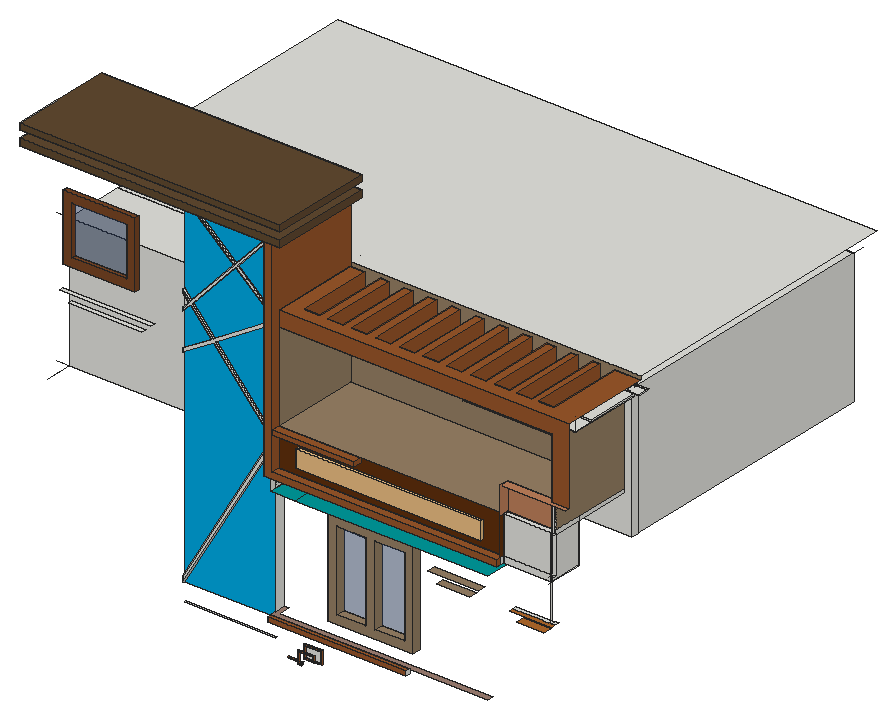
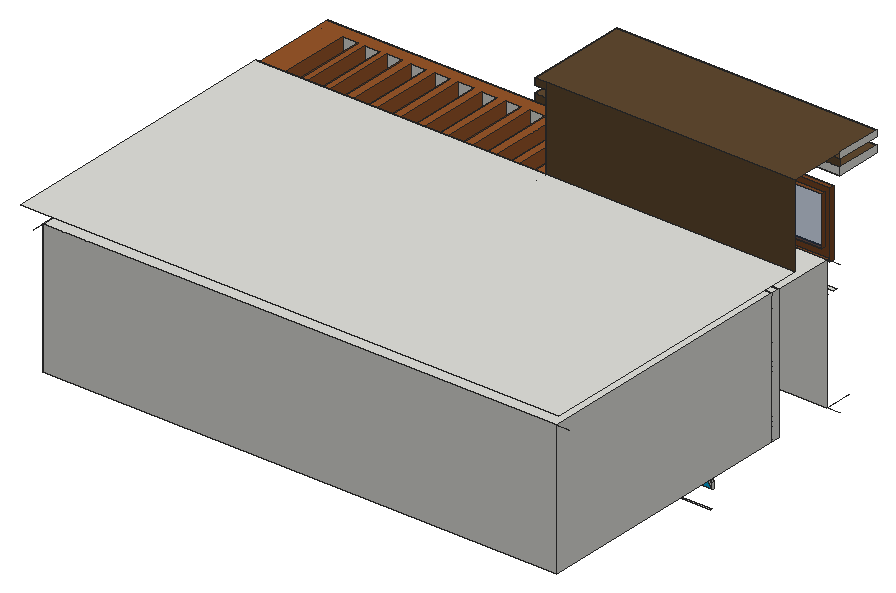
# SketchUp Ruby script. Lengths in inches.
U = 1.inch
M = Sketchup.active_model
def pt(a) = Geom::Point3d.new(a.map { |v| v * U })
def face(e, loops, mat)
  f = e.add_face(loops[0].map { |a| pt(a) })
  loops[1..].each { |l| e.add_face(l.map { |a| pt(a) }).erase! }
  f.material = f.back_material = mat if mat
  f
end
# faces: each face lists its corners as indices into pts; further lists are holes
def faces(e, pts, list, mat = nil) = list.each { |f| face(e, (f[0].is_a?(Array) ? f : [f]).map { |l| l.map { |i| pts[i] } }, mat) }
# xy, xz, yz: faces in a plane at the given z, y or x. An outline is a flat list of corners, or four numbers for a rectangle; further outlines are holes
def ring(l) = l.size == 4 ? [[l[0], l[1]], [l[2], l[1]], [l[2], l[3]], [l[0], l[3]]] : l.each_slice(2).to_a
def flat(e, list, mat, &to3) = list.each { |f| face(e, (f[0].is_a?(Array) ? f : [f]).map { |l| ring(l).map { |u, v| to3.(u, v) } }, mat) }
def xy(e, z, list, mat = nil) = flat(e, list, mat) { |x, y| [x, y, z] }
def xz(e, y, list, mat = nil) = flat(e, list, mat) { |x, z| [x, y, z] }
def yz(e, x, list, mat = nil) = flat(e, list, mat) { |y, z| [x, y, z] }
def lines(e, pts, list) = list.each { |a, b| e.add_line(pt(pts[a]), pt(pts[b])) }
# prism: a flat outline (further loops are holes) pulled along v
def prism(e, loops, v, mat = nil)
  f = face(e, loops, mat); d = Geom::Vector3d.new(v.map { |x| x * U })
  f.pushpull(f.normal.samedirection?(d) ? d.length : -d.length)
end
def box(e, o, s, mat = nil) = prism(e, [[o, [o[0] + s[0], o[1], o[2]], [o[0] + s[0], o[1] + s[1], o[2]], [o[0], o[1] + s[1], o[2]]]], [0, 0, s[2]], mat)
def at(x, y, z, deg = 0) = Geom::Transformation.translation(pt([x, y, z])) * Geom::Transformation.rotation(ORIGIN, Z_AXIS, deg.degrees)
def axes(o, x, y, z) = Geom::Transformation.new([*x, 0, *y, 0, *z, 0, *pt(o).to_a, 1])
def part(name) = M.definitions.add(name)
# library, detail: a bought-in or finely detailed component or shape, given as its bounding box
def library(name, o, s) = part(name).tap { |d| box(d.entities, o, s) }
def detail(e, o, s) = box(e.add_group.entities, o, s)
def put(e, d, t, mat = nil) = e.add_instance(d, t).tap { |i| i.material = mat if mat }
def group(e, t, mat = nil) = e.add_group.tap { |g| g.transformation = t; g.material = mat if mat }.entities
root = M.entities
M.materials.add("Niraj_Shoe_Sole").color = [96, 73, 48]
M.materials.add("Niraj_Skin").color = [158, 128, 115]
M.materials.add("[0035_Tan]").color = [150, 128, 100]
M.materials.add("[0043_SaddleBrown]").color = [96, 48, 13]
M.materials.add("[0083_DarkTurquoise]").color = [0, 153, 155]
M.materials.add("[0097_DeepSkyBlue]").color = [0, 169, 226]
M.materials.add("[0097_DeepSkyBlue]1").color = [0, 171, 229]
M.materials.add("[Basketweave]").color = [230, 230, 230]
M.materials.add("[Translucent Glass Blue]").color = [40, 60, 96]
M.materials["[Translucent Glass Blue]"].alpha = 0.5
M.materials.add("[Wood Bamboo]").color = [177, 105, 43]
M.materials.add("[Wood Cherry Original]").color = [152, 86, 42]
M.materials.add("[Wood Veneer 01]").color = [120, 70, 37]
M.materials.add("[Wood Veneer 02]").color = [190, 128, 91]
c1 = library("NAKSHA MART",[0.95,0,0],[104.73,9.95,1])
xy(root,148.76,[[191.85,117,194.8,118]],"[Wood Cherry Original]")
xy(root,149.21,[[192.49,117,194.8,118]],"[Wood Cherry Original]")
xy(root,150.16,[[185.22,117,191.85,118],[192.49,117,194.8,118]],"[Wood Cherry Original]")
xy(root,150.73,[[184.65,117,191.85,118],[192.49,117,195.37,118]],"[Wood Cherry Original]")
xy(root,153.79,[[196.34,117,203.17,118],[203.17,117,208.53,118]],"[Wood Cherry Original]")
xy(root,154.4,[[196.95,117,202.56,118],[203.17,117,207.92,118]],"[Wood Cherry Original]")
xy(root,156.27,[[106.63,122.375,171.63,123.3125]])
xy(root,157.02,[[192.49,117,196.95,118],[196.95,117,202.56,118]],"[Wood Cherry Original]")
xy(root,157.63,[[191.85,117,196.34,118],[196.95,117,203.17,118]],"[Wood Cherry Original]")
xy(root,162.4375,[[196.95,117,207.92,118]],"[Wood Cherry Original]")
xy(root,163.04,[[196.34,117,208.53,118]],"[Wood Cherry Original]")
xy(root,169.5625,[[171.63,115,270.57,118]],"[Wood Cherry Original]")
xy(root,170.25,[[198.26,136,258.45,142]])
xy(root,172.875,[[171.63,118,326.57,118,326.57,122.125,175.07,122.125,175.07,130,171.63,130]],"Niraj_Skin")
xy(root,172.875,[[171.63,115,270.57,118]],"[Wood Cherry Original]")
xy(root,176.25,[[204.26,136,225.35,142],[231.35,136,252.45,142]],"[0035_Tan]")
xy(root,220.875,[[275.26,136,299.26,142]],"[0035_Tan]")
xy(root,226.875,[[269.26,136,305.26,142]],"[0035_Tan]")
xy(root,233,[[204.26,136,225.35,142],[231.35,136,252.45,142]],"[0035_Tan]")
xy(root,233.83,[[351.89,112,371.22,118]],"[Wood Bamboo]")
xy(root,239,[[198.26,136,258.45,142]],"[0035_Tan]")
xy(root,239.26,[[346.46,115,372,118],[372,115,374.5,118],[374.5,115,376.65,118]])
xy(root,239.26,[[346.46,112,376.65,115]],"[Wood Bamboo]")
xy(root,251.8,[[171.63,130,189.04,142]])
xy(root,251.8,[[171.63,118,189.04,130],[189.04,118,326.57,142]],"[0083_DarkTurquoise]")
xy(root,264,[[171.63,118,337.38,142],[337.38,118,337.94,142],[337.94,118,371.25,142],[371.25,118,372,142],[9,185.375,375,190.9375],
  [9,190.9375,375,191.0625]])
xy(root,264,[[171.63,112,337.38,118]],"[Wood Cherry Original]")
xy(root,268.5,[[177.19,112,337.38,118]],"[Wood Cherry Original]")
xy(root,292.26,[[177.19,112,236,118]],"[Wood Cherry Original]")
xy(root,292.65,[[337.38,121.62,337.94,142],[371.25,121.62,371.25,142,337.38,142,337.38,182.0625,372,182.0625,372,121.62],[337.94,121.62,371.25,142]])
xy(root,295.34,[[337.38,118,337.94,121.62],[337.94,118,371.25,121.62],[371.25,118,372,121.62]])
xy(root,295.34,[[177.19,118,337.38,118,337.38,121.62,372,121.62,372,182.0625,177.19,182.0625]],"[0035_Tan]")
xy(root,295.34,[[177.19,112,236,118]],"[Wood Cherry Original]")
xy(root,310.87,[[257.29,182.0625,340.41,185.375]])
xy(root,314.9,[[337.38,115,384,115,384,118,372,118,372,121.62,337.38,121.62]],"[Wood Veneer 02]")
xy(root,319.95,[[26.53,119.375,78.96,122.375]])
xy(root,326.3125,[[20.16,119.375,85.33,122.375]])
xy(root,343.6,[[22.76,119.375,74.01,122.375]],"[Wood Veneer 01]")
xy(root,348.68,[[257.29,182.0625,340.41,185.375]])
xy(root,349.76,[[28.92,119.375,67.85,122.375]],"[Wood Veneer 01]")
xy(root,358.625,[[372,127.53,381.34,142],[372,127.53,381.34,179.66],[9,142,177.19,185.375],[372,182.0625,375,185.375],[375,182.0625,382.75,189.21],
  [9,185.375,177.19,190.9375],[177.19,185.375,177.19,190.9375,373.3125,190.9375,373.3125,189.21,372,189.21,372,185.375],[372,185.375,375,189.21],[373.3125,189.21,375,190.9375],[375,189.21,382.75,191.0625],
  [9,190.9375,177.19,191.0625],[177.19,190.9375,372,191.0625],[372,190.9375,373.3125,191.0625],[373.3125,190.9375,375,191.0625],[9,191.0625,9,382.875,375,382.875,375,191.0625,372,191.0625,372,191.1875,177.19,191.1875,177.19,191.0625],
  [177.19,191.0625,372,191.1875]])
xy(root,358.625,[[177.19,118,177.19,181.83,187.9,181.83,187.9,127.72,198.78,127.72,198.78,181.83,204.84,181.83,204.84,127.53,215.72,127.53,215.72,181.83,221.78,181.83,221.78,127.53,232.65,127.53,232.65,181.83,238.72,181.83,238.72,127.53,249.59,127.53,249.59,181.83,255.65,181.83,255.65,127.53,266.53,127.53,266.53,181.83,272.59,181.83,272.59,127.53,283.47,127.53,283.47,181.83,289.53,181.83,289.53,127.53,300.4,127.53,300.4,181.83,306.47,181.83,306.47,127.53,317.34,127.53,317.34,181.83,323.4,181.83,323.4,127.53,334.28,127.53,334.28,181.83,339.09,181.83,339.09,127.53,349.97,127.53,349.97,181.83,354.78,181.83,354.78,127.53,365.65,127.53,365.65,181.83,372,181.83,372,118]],"[Wood Cherry Original]")
xy(root,358.9375,[[370.47,127.53,381.34,179.66],[365.65,181.83,372,190.89],[372,182.0625,373.3125,189.21]])
xy(root,359.1875,[[171.63,118,177.19,142],[373.3125,182.0625,382.75,189.21]])
xy(root,359.625,[[370.47,127.53,372,179.66]])
xy(root,360.375,[[372,142,381.34,179.66]])
xy(root,361.5,[[171.63,118,177.19,142]])
xy(root,369.0625,[[177.19,118,384,118,384,182.0625,375,182.0625,375,181.83,365.65,181.83,365.65,127.53,354.78,127.53,354.78,181.83,349.97,181.83,349.97,127.53,339.09,127.53,339.09,181.83,334.28,181.83,334.28,127.53,323.4,127.53,323.4,181.83,317.34,181.83,317.34,127.53,306.47,127.53,306.47,181.83,300.4,181.83,300.4,127.53,289.53,127.53,289.53,181.83,283.47,181.83,283.47,127.53,272.59,127.53,272.59,181.83,266.53,181.83,266.53,127.53,255.65,127.53,255.65,181.83,249.59,181.83,249.59,127.53,238.72,127.53,238.72,181.83,232.65,181.83,232.65,127.53,221.78,127.53,221.78,181.83,215.72,181.83,215.72,127.53,204.84,127.53,204.84,181.83,198.78,181.83,198.78,127.72,187.9,127.72,187.9,181.83,177.19,181.83]],"[Wood Cherry Original]")
xy(root,371.75,[[0,182.0625,384,391.875]])
xy(root,384.9375,[[28.92,119.375,67.85,122.375]],"[Wood Veneer 01]")
xy(root,391.1,[[22.76,119.375,74.01,122.375]],"[Wood Veneer 01]")
xy(root,415.46,[[171.63,112,177.19,118],[171.63,118,177.19,142],[106.63,121.375,106.63,122.375,0,122.375,0,142,171.63,142,171.63,122.375,109.24,122.375,109.24,121.375]])
xy(root,415.46,[[0,109.5625,0,122.375,106.63,122.375,106.63,121.375,109.24,121.375,109.24,122.375,171.63,122.375,171.63,112,177.19,112,177.19,182.0625,185.19,182.0625,185.19,109.5625]],"Niraj_Shoe_Sole")
xy(root,420.59,[[0,109.5625,185.19,109.5625,185.19,182.0625,177.19,182.0625,177.19,142,0,142]],"Niraj_Shoe_Sole")
xy(root,425.72,[[0,109.5625,0,142,177.19,142,177.19,182.0625,185.19,182.0625,185.19,109.5625]],"Niraj_Shoe_Sole")
xy(root,430.21,[[0,109.5625,185.19,182.0625]],"Niraj_Shoe_Sole")
xz(root,109.5625,[[0,415.46,185.19,420.59],[0,425.72,185.19,430.21]],"Niraj_Shoe_Sole")
xz(root,112,[[171.63,264,337.38,264,337.38,268.5,177.19,268.5,177.19,415.46,171.63,415.46],[177.19,292.26,236,295.34]],"[Wood Cherry Original]")
xz(root,115,[[171.63,169.5625,270.57,172.875]],"[Wood Cherry Original]")
xz(root,117,[[191.85,150.73,192.49,150.73,192.49,157.02,202.56,157.02,202.56,154.4,196.95,154.4,196.95,157.02,196.34,157.01,196.34,153.79,203.17,153.79,203.17,157.63,191.85,157.63],[203.17,153.79,208.53,153.79,208.53,163.04,196.34,163.04,196.34,157.63,196.95,157.63,196.95,162.4375,207.92,162.4375,207.92,154.4,203.17,154.4]],"[Wood Cherry Original]")
xz(root,118,[[192.49,149.21,194.8,150.16],[196.95,154.4,202.56,157.02],[203.17,154.4,207.92,154.4,207.92,162.4375,196.95,162.4375,196.95,157.63,203.17,157.63],[171.63,169.5625,270.57,172.875],[371.25,239.26,372,264],
  [171.63,264,171.63,359.1875,177.19,359.1875,177.19,268.5,337.38,268.5,337.38,264],[337.38,264,337.94,268.5],[337.94,264,371.25,268.5],[371.25,264,372,268.5],[337.38,268.5,337.94,295.34],
  [337.94,268.5,371.25,295.34],[371.25,268.5,372,295.34],[372,268.5,374.5,295.34],[177.19,292.26,236,293.14],[177.19,293.14,236,295.34],
  [372,295.34,373.19,314.9],[171.63,359.1875,177.19,361.5]])
xz(root,118,[[177.19,268.5,337.38,268.5,337.38,295.34,236,295.34,236,292.26,177.19,292.26]],"[0043_SaddleBrown]")
xz(root,118,[[372,314.9,384,314.9,384,369.0625,177.19,369.0625,177.19,358.625,372,358.625]],"[Wood Cherry Original]")
xz(root,119.375,[[[22.76,343.6,74.01,391.1],[28.92,349.76,67.85,384.9375]]],"[Wood Veneer 01]")
xz(root,121.375,[[106.63,169.15,171.63,280.38,171.63,283.38,129.8125,330.53,171.63,356.59,171.63,359.1875,128.36,332.17,113.11,349.37,144.1,383.02,171.63,359.1875,171.63,361.5,145.27,384.3,171.63,412.93,171.63,415.46,144.03,385.37,109.24,415.46,106.63,415.46,142.86,384.09,112.08,350.53,106.63,356.67,106.63,353.72,110.75,349.07,106.63,344.58,106.63,342.33,111.77,347.92,126.66,331.12,106.63,318.61,106.63,316.08,128.12,329.47,169.73,282.52,106.63,173.48]])
xz(root,121.62,[[337.38,292.65,337.94,295.34],[337.94,292.65,371.25,295.34],[371.25,292.65,372,295.34]])
xz(root,121.62,[[337.38,295.34,372,314.9]],"[Wood Veneer 02]")
xz(root,122.375,[[106.63,344.58,110.75,349.07,106.63,353.72]])
xz(root,122.375,[[106.63,173.48,169.73,282.52,128.12,329.47,106.63,316.08],[171.63,283.38,171.63,356.59,129.8125,330.53],[106.63,318.61,126.66,331.12,111.77,347.92,106.63,342.33],[128.36,332.17,171.63,359.1875,144.1,383.02,113.11,349.37],[112.08,350.53,142.86,384.09,106.63,415.46,106.63,356.67],
  [171.63,361.5,171.63,412.93,145.27,384.3],[144.03,385.37,171.63,415.46,109.24,415.46]],"[0097_DeepSkyBlue]")
xz(root,122.375,[[106.63,169.15,171.63,169.15,171.63,280.38]],"[0097_DeepSkyBlue]1")
xz(root,122.375,[[28.92,349.76,67.85,384.9375]],"[Translucent Glass Blue]")
xz(root,127.53,[[204.84,358.625,215.72,358.9375],[221.78,358.625,232.65,358.9375],[238.72,358.625,249.59,358.9375],[255.65,358.625,266.53,358.9375],[272.59,358.625,283.47,358.9375],
  [289.53,358.625,300.4,358.9375],[306.47,358.625,317.34,358.9375],[323.4,358.625,334.28,358.9375],[339.09,358.625,349.97,358.9375],[354.78,358.625,365.65,358.9375],
  [372,358.625,381.34,358.9375],[204.84,358.9375,215.72,369.0625],[221.78,358.9375,232.65,369.0625],[238.72,358.9375,249.59,369.0625],[255.65,358.9375,266.53,369.0625],
  [272.59,358.9375,283.47,369.0625],[289.53,358.9375,300.4,369.0625],[306.47,358.9375,317.34,369.0625],[323.4,358.9375,334.28,369.0625],[339.09,358.9375,349.97,369.0625],
  [354.78,358.9375,365.65,369.0625],[370.47,358.9375,372,359.625]])
xz(root,127.72,[[187.9,358.625,198.78,358.9375],[187.9,358.9375,198.78,369.0625]])
xz(root,136,[[[198.26,170.25,258.45,239],[204.26,176.25,225.35,233],[231.35,176.25,252.45,233]]],"[0035_Tan]")
xz(root,142,[[9,264,171.63,358.625],[337.38,264,337.94,292.65],[337.94,264,371.25,292.65],[171.63,358.625,177.19,359.1875],[372,358.625,381.34,360.375],
  [171.63,359.1875,177.19,361.5],[0,415.46,171.63,420.59],[171.63,415.46,177.19,420.59]])
xz(root,142,[[0,420.59,177.19,425.72]],"Niraj_Shoe_Sole")
xz(root,142,[[204.26,176.25,225.35,233],[231.35,176.25,252.45,233]],"[Translucent Glass Blue]")
xz(root,179.66,[[372,358.625,381.34,358.9375],[370.47,358.9375,372,359.625],[372,358.9375,381.34,360.375]])
xz(root,181.83,[[177.19,358.625,187.9,358.9375],[198.78,358.625,204.84,358.9375],[215.72,358.625,221.78,358.9375],[232.65,358.625,238.72,358.9375],[249.59,358.625,255.65,358.9375],
  [266.53,358.625,272.59,358.9375],[283.47,358.625,289.53,358.9375],[300.4,358.625,306.47,358.9375],[317.34,358.625,323.4,358.9375],[334.28,358.625,339.09,358.9375],
  [349.97,358.625,354.78,358.9375],[365.65,358.625,372,358.9375],[372,358.625,372,358.9375,365.65,358.9375,365.65,369.0625,375,369.0625,375,358.625],[177.19,358.9375,187.9,369.0625],[198.78,358.9375,204.84,369.0625],
  [215.72,358.9375,221.78,369.0625],[232.65,358.9375,238.72,369.0625],[249.59,358.9375,255.65,369.0625],[266.53,358.9375,272.59,369.0625],[283.47,358.9375,289.53,369.0625],
  [300.4,358.9375,306.47,369.0625],[317.34,358.9375,323.4,369.0625],[334.28,358.9375,339.09,369.0625],[349.97,358.9375,354.78,369.0625]])
xz(root,182.0625,[[337.38,292.65,372,295.34],[372,358.625,375,358.9375],[375,358.625,382.75,358.9375],[373.3125,358.9375,375,359.1875],[375,358.9375,382.75,359.1875]])
xz(root,182.0625,[[0,371.75,177.19,430.21],[177.19,415.46,185.19,420.59],[177.19,425.72,185.19,430.21]],"Niraj_Shoe_Sole")
xz(root,182.0625,[[[177.19,295.34,372,295.34,372,358.9375,373.3125,358.9375,373.3125,359.1875,375,359.1875,375,369.0625,384,369.0625,384,371.75,177.19,371.75],[257.29,310.87,340.41,348.68]]],"[0035_Tan]")
xz(root,185.375,[[[9,264,375,358.625],[257.29,310.87,340.41,348.68]]])
xz(root,189.21,[[372,358.625,373.3125,358.9375],[373.3125,358.625,382.75,358.9375],[373.3125,358.9375,382.75,359.1875]])
xz(root,190.9375,[[9,264,375,358.625]],"[Basketweave]")
xz(root,191.0625,[[9,264,375,358.625]])
xz(root,382.875,[[9,264,375,358.625]])
yz(root,0,[[109.5625,415.46,142,420.59],[109.5625,425.72,142,430.21]])
yz(root,9,[[185.375,264,190.9375,358.625],[190.9375,264,191.0625,358.625],[191.0625,264,382.875,358.625]])
yz(root,22.76,[[119.375,343.6,122.375,391.1]],"[Wood Veneer 01]")
yz(root,28.92,[[119.375,349.76,122.375,384.9375]],"[Wood Veneer 01]")
yz(root,67.85,[[119.375,349.76,122.375,384.9375]],"[Wood Veneer 01]")
yz(root,74.01,[[119.375,343.6,122.375,391.1]],"[Wood Veneer 01]")
yz(root,106.63,[[121.375,169.15,122.375,173.48],[121.375,316.08,122.375,318.61],[121.375,342.33,122.375,344.58],[121.375,353.72,122.375,356.67]])
yz(root,171.63,[[122.375,172.875,130,251.8],[118,251.8,122.375,264],[122.375,251.8,142,264],[118,264,118,359.1875,121.375,359.1875,121.375,356.59,122.375,356.59,122.375,283.38,121.375,283.38,121.375,280.38,122.375,280.38,122.375,264],[122.375,264,122.375,280.38,121.375,280.38,121.375,283.38,122.375,283.38,122.375,356.59,121.375,356.59,121.375,358.625,142,358.625,142,264],
  [112,295.34,118,295.46],[121.375,358.625,142,359.1875],[118,359.1875,121.375,361.5],[121.375,359.1875,142,361.5],[118,361.5,118,415.46,121.375,415.46,121.375,412.93,122.375,412.93,122.375,361.5],
  [122.375,361.5,122.375,412.93,121.375,412.93,121.375,415.46,142,415.46,142,361.5]])
yz(root,171.63,[[115,169.5625,118,172.875],[112,264,118,295.34],[112,295.46,118,415.46]],"[Wood Cherry Original]")
yz(root,177.19,[[112,292.26,118,293.14],[112,293.14,118,295.34],[118,358.625,142,358.9375],[142,358.625,181.83,358.9375],[118,358.9375,142,359.1875],
  [142,358.9375,181.83,369.0625],[118,359.1875,142,361.5],[118,361.5,142,369.0625],[142,415.46,182.0625,420.59]])
yz(root,177.19,[[142,420.59,182.0625,425.72]],"Niraj_Shoe_Sole")
yz(root,177.19,[[118,295.34,182.0625,358.625]],"[0035_Tan]")
yz(root,177.19,[[112,268.5,118,292.26],[112,295.34,118,295.34,118,369.0625,181.83,369.0625,181.83,358.625,182.0625,358.625,182.0625,415.46,112,415.46]],"[Wood Cherry Original]")
yz(root,185.19,[[109.5625,415.46,182.0625,420.59],[109.5625,425.72,182.0625,430.21]],"Niraj_Shoe_Sole")
yz(root,187.9,[[127.72,358.625,181.83,369.0625]],"[Wood Cherry Original]")
yz(root,191.85,[[117,148.76,118,150.16],[117,150.73,118,157.02],[117,157.02,118,157.63]],"[Wood Cherry Original]")
yz(root,192.49,[[117,149.21,118,150.16],[117,150.73,118,157.02]],"[Wood Cherry Original]")
yz(root,194.8,[[117,149.21,118,150.16]],"[Wood Cherry Original]")
yz(root,196.34,[[117,153.79,118,157.01],[117,157.63,118,163.04]],"[Wood Cherry Original]")
yz(root,196.95,[[117,154.4,118,157.02],[117,157.63,118,162.4375]],"[Wood Cherry Original]")
yz(root,198.26,[[136,170.25,142,239]],"[0035_Tan]")
yz(root,198.78,[[127.72,358.625,181.83,369.0625]],"[Wood Cherry Original]")
yz(root,202.56,[[117,154.4,118,157.02]],"[Wood Cherry Original]")
yz(root,203.17,[[117,154.4,118,157.63]],"[Wood Cherry Original]")
yz(root,204.26,[[136,176.25,142,233]],"[0035_Tan]")
yz(root,204.84,[[127.53,358.625,181.83,369.0625]],"[Wood Cherry Original]")
yz(root,207.92,[[117,154.4,118,162.4375]],"[Wood Cherry Original]")
yz(root,208.53,[[117,153.79,118,163.04]],"[Wood Cherry Original]")
yz(root,215.72,[[127.53,358.625,181.83,369.0625]],"[Wood Cherry Original]")
yz(root,221.78,[[127.53,358.625,181.83,369.0625]],"[Wood Cherry Original]")
yz(root,225.35,[[136,176.25,142,233]],"[0035_Tan]")
yz(root,231.35,[[136,176.25,142,233]],"[0035_Tan]")
yz(root,232.65,[[127.53,358.625,181.83,369.0625]],"[Wood Cherry Original]")
yz(root,236,[[112,292.26,118,295.34]],"[Wood Cherry Original]")
yz(root,238.72,[[127.53,358.625,181.83,369.0625]],"[Wood Cherry Original]")
yz(root,249.59,[[127.53,358.625,181.83,369.0625]],"[Wood Cherry Original]")
yz(root,252.45,[[136,176.25,142,233]],"[0035_Tan]")
yz(root,255.65,[[127.53,358.625,181.83,369.0625]],"[Wood Cherry Original]")
yz(root,257.29,[[182.0625,310.87,185.375,348.68]])
yz(root,258.45,[[136,170.25,142,239]],"[0035_Tan]")
yz(root,266.53,[[127.53,358.625,181.83,369.0625]],"[Wood Cherry Original]")
yz(root,270.57,[[115,169.5625,118,172.875]])
yz(root,272.59,[[127.53,358.625,181.83,369.0625]],"[Wood Cherry Original]")
yz(root,283.47,[[127.53,358.625,181.83,369.0625]],"[Wood Cherry Original]")
yz(root,289.53,[[127.53,358.625,181.83,369.0625]],"[Wood Cherry Original]")
yz(root,300.4,[[127.53,358.625,181.83,369.0625]],"[Wood Cherry Original]")
yz(root,306.47,[[181.83,358.625,182.0625,361.625]])
yz(root,306.47,[[127.53,358.625,181.83,369.0625]],"[Wood Cherry Original]")
yz(root,317.34,[[181.83,358.625,182.0625,361.625]])
yz(root,317.34,[[127.53,358.625,181.83,369.0625]],"[Wood Cherry Original]")
yz(root,323.4,[[127.53,358.625,181.83,369.0625]],"[Wood Cherry Original]")
yz(root,334.28,[[127.53,358.625,181.83,369.0625]],"[Wood Cherry Original]")
yz(root,337.38,[[115,264,118,268.5],[118,264,118,295.34,121.62,295.34,121.62,292.65,142,292.65,142,264]])
yz(root,337.38,[[115,268.5,118,295.34]],"[0043_SaddleBrown]")
yz(root,337.38,[[112,264,115,268.5]],"[Wood Cherry Original]")
yz(root,337.38,[[115,295.34,121.62,314.9]],"[Wood Veneer 02]")
yz(root,337.94,[[118,264,118,295.34,121.62,295.34,121.62,292.65,142,292.65,142,264]])
yz(root,339.09,[[127.53,358.625,181.83,369.0625]],"[Wood Cherry Original]")
yz(root,340.41,[[182.0625,310.87,185.375,348.68]])
yz(root,349.97,[[127.53,358.625,181.83,369.0625]],"[Wood Cherry Original]")
yz(root,354.78,[[127.53,358.625,181.83,369.0625]],"[Wood Cherry Original]")
yz(root,365.65,[[181.83,358.9375,190.89,369.0625]])
yz(root,365.65,[[127.53,358.625,181.83,369.0625]],"[Wood Cherry Original]")
yz(root,370.47,[[127.53,358.9375,179.66,359.625]])
yz(root,371.25,[[118,264,142,264,142,292.65,121.62,292.65,121.62,295.34,118,295.34]])
yz(root,372,[[121.62,292.65,142,295.34],[142,292.65,182.0625,295.34],[118,295.34,121.62,308.28],[118,308.28,121.62,314.9],[127.53,358.625,142,359.625],
  [142,358.625,179.66,359.625],[181.83,358.625,182.0625,358.9375],[182.0625,358.625,189.21,358.9375],[142,359.625,179.66,360.375]])
yz(root,372,[[121.62,295.34,121.62,314.9,118,314.9,118,358.625,182.0625,358.625,182.0625,295.34]],"[0035_Tan]")
yz(root,373.3125,[[182.0625,358.9375,189.21,359.1875]])
yz(root,375,[[185.375,264,190.9375,358.625],[190.9375,264,191.0625,358.625],[191.0625,264,382.875,358.625],[181.83,358.625,182.0625,369.0625]])
yz(root,381.34,[[127.53,358.625,142,358.9375],[142,358.625,179.66,358.9375],[142,358.9375,179.66,360.375]])
yz(root,382.75,[[182.0625,358.625,189.21,359.1875]])
p = [[196.95,118,157.02],[196.34,118,157.01],[196.34,117,157.01],[196.95,117,157.02],[106.63,122.375,169.15],[171.63,122.375,280.38],
  [171.63,121.375,280.38],[106.63,121.375,169.15],[169.73,122.375,282.52],[106.63,122.375,173.48],[106.63,121.375,173.48],[169.73,121.375,282.52],
  [128.12,122.375,329.47],[128.12,121.375,329.47],[171.63,122.375,283.38],[129.8125,122.375,330.53],[129.8125,121.375,330.53],[171.63,121.375,283.38],
  [106.63,122.375,316.08],[106.63,121.375,316.08],[126.66,122.375,331.12],[106.63,122.375,318.61],[106.63,121.375,318.61],[126.66,121.375,331.12],
  [171.63,122.375,356.59],[171.63,121.375,356.59],[111.77,122.375,347.92],[111.77,121.375,347.92],[128.36,122.375,332.17],[113.11,122.375,349.37],
  [113.11,121.375,349.37],[128.36,121.375,332.17],[171.63,122.375,359.1875],[171.63,121.375,359.1875],[106.63,122.375,342.33],[106.63,121.375,342.33],
  [110.75,122.375,349.07],[106.63,122.375,344.58],[106.63,121.375,344.58],[110.75,121.375,349.07],[106.63,122.375,353.72],[106.63,121.375,353.72],
  [144.1,122.375,383.02],[144.1,121.375,383.02],[112.08,122.375,350.53],[106.63,122.375,356.67],[106.63,121.375,356.67],[112.08,121.375,350.53],
  [142.86,122.375,384.09],[142.86,121.375,384.09],[171.63,122.375,361.5],[145.27,122.375,384.3],[145.27,121.375,384.3],[171.63,121.375,361.5],
  [106.63,122.375,415.46],[106.63,121.375,415.46],[171.63,122.375,412.93],[171.63,121.375,412.93],[144.03,122.375,385.37],[109.24,122.375,415.46],
  [109.24,121.375,415.46],[144.03,121.375,385.37],[171.63,122.375,415.46],[171.63,121.375,415.46],[372,142,264],[372,142,292.65],
  [177.19,182.0625,295.34],[177.19,191.0625,295.34],[337.38,182.0625,295.34],[337.38,191.0625,295.34],[198.78,127.53,361.625],[198.78,127.53,358.625],
  [187.34,179.66,361.625],[187.34,179.66,358.625],[187.34,127.53,361.625],[187.34,127.53,358.625],[199.9,127.53,361.625],[199.9,127.53,358.625],
  [199.9,179.66,361.625],[199.9,179.66,358.625],[372,118,358.625],[372,118,358.9375],[381.34,127.53,358.9375],[381.34,127.53,369.0625],
  [177.19,191.1875,358.625],[177.19,191.1875,371.75],[370.47,179.66,358.625],[370.47,179.66,358.9375],[370.47,127.53,358.625],[370.47,127.53,358.9375],
  [375,382.875,358.625],[375,391.875,358.625],[9,382.875,358.625],[0,382.875,358.625],[9,142,358.625],[0,142,358.625],
  [337.38,142,292.65],[337.38,142,295.34],[9,142,264],[9,122.375,264],[0,142,264],[374.5,118,295.34],
  [374.5,115,295.34],[374.5,118,268.5],[374.5,115,268.5],[372,118,268.5],[372,115,268.5],[373.19,118,295.34],
  [373.19,115,295.34],[372,118,264],[372,115,264]]
faces(root,p,[[0,1,2,3],[4,5,6,7],[8,9,10,11],[12,8,11,13],[14,15,16,17],[18,12,13,19],[20,21,22,23],[15,24,25,16],
  [26,20,23,27],[28,29,30,31],[32,28,31,33],[34,26,27,35],[36,37,38,39],[40,36,39,41],[29,42,43,30],[44,45,46,47],
  [48,44,47,49],[42,32,33,43],[50,51,52,53],[54,48,49,55],[51,56,57,52],[58,59,60,61],[62,58,61,63]])
lines(root,p,[[64,65],[66,67],[68,69],[70,71],[72,73],[74,75],[76,77],[78,79],[80,81],[82,83],[84,85],[86,87],
  [88,89],[90,91],[92,93],[94,95],[96,97],[98,99],[98,100],[101,102],[103,104],[105,106],[107,108],[109,110]])
put(root,c1,axes([190.41,118,274.1875],[1.2543,0,0],[0,0,1.2543],[0,-2.22011,0]))
